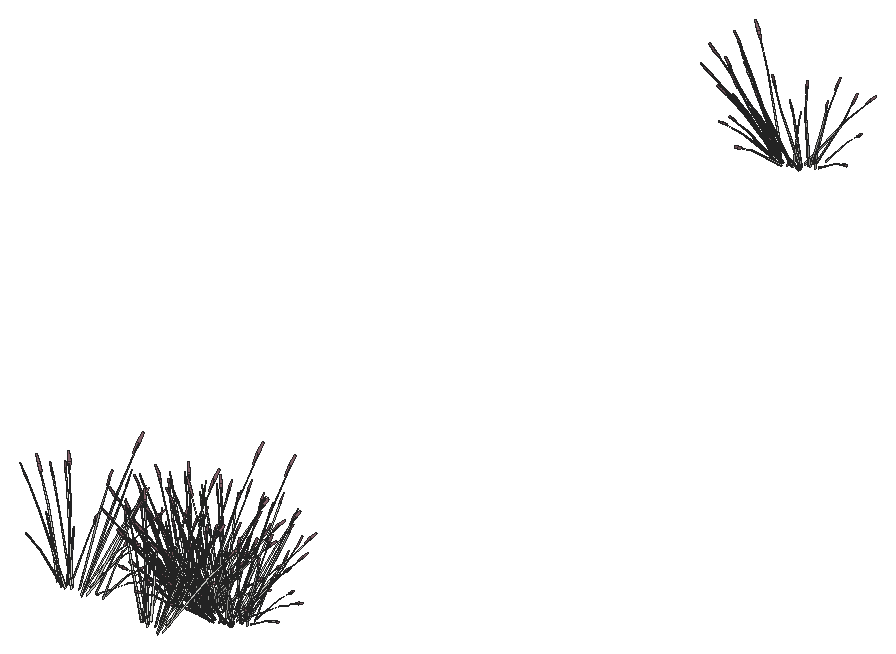
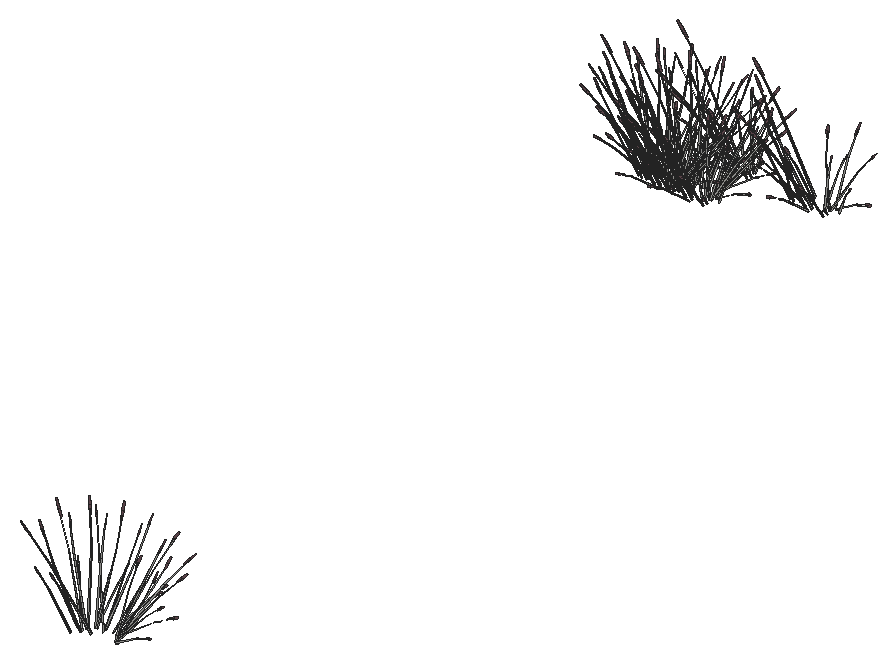
# SketchUp Ruby script. Lengths in inches.
U = 1.inch
M = Sketchup.active_model
def pt(a) = Geom::Point3d.new(a.map { |v| v * U })
def face(e, loops, mat)
  f = e.add_face(loops[0].map { |a| pt(a) })
  loops[1..].each { |l| e.add_face(l.map { |a| pt(a) }).erase! }
  f.material = f.back_material = mat if mat
  f
end
# faces: each face lists its corners as indices into pts; further lists are holes
def faces(e, pts, list, mat = nil) = list.each { |f| face(e, (f[0].is_a?(Array) ? f : [f]).map { |l| l.map { |i| pts[i] } }, mat) }
# xy, xz, yz: faces in a plane at the given z, y or x. An outline is a flat list of corners, or four numbers for a rectangle; further outlines are holes
def ring(l) = l.size == 4 ? [[l[0], l[1]], [l[2], l[1]], [l[2], l[3]], [l[0], l[3]]] : l.each_slice(2).to_a
def flat(e, list, mat, &to3) = list.each { |f| face(e, (f[0].is_a?(Array) ? f : [f]).map { |l| ring(l).map { |u, v| to3.(u, v) } }, mat) }
def xy(e, z, list, mat = nil) = flat(e, list, mat) { |x, y| [x, y, z] }
def xz(e, y, list, mat = nil) = flat(e, list, mat) { |x, z| [x, y, z] }
def yz(e, x, list, mat = nil) = flat(e, list, mat) { |y, z| [x, y, z] }
def lines(e, pts, list) = list.each { |a, b| e.add_line(pt(pts[a]), pt(pts[b])) }
# prism: a flat outline (further loops are holes) pulled along v
def prism(e, loops, v, mat = nil)
  f = face(e, loops, mat); d = Geom::Vector3d.new(v.map { |x| x * U })
  f.pushpull(f.normal.samedirection?(d) ? d.length : -d.length)
end
def box(e, o, s, mat = nil) = prism(e, [[o, [o[0] + s[0], o[1], o[2]], [o[0] + s[0], o[1] + s[1], o[2]], [o[0], o[1] + s[1], o[2]]]], [0, 0, s[2]], mat)
def at(x, y, z, deg = 0) = Geom::Transformation.translation(pt([x, y, z])) * Geom::Transformation.rotation(ORIGIN, Z_AXIS, deg.degrees)
def axes(o, x, y, z) = Geom::Transformation.new([*x, 0, *y, 0, *z, 0, *pt(o).to_a, 1])
def part(name) = M.definitions.add(name)
# library, detail: a bought-in or finely detailed component or shape, given as its bounding box
def library(name, o, s) = part(name).tap { |d| box(d.entities, o, s) }
def detail(e, o, s) = box(e.add_group.entities, o, s)
def put(e, d, t, mat = nil) = e.add_instance(d, t).tap { |i| i.material = mat if mat }
def group(e, t, mat = nil) = e.add_group.tap { |g| g.transformation = t; g.material = mat if mat }.entities
root = M.entities
M.materials.add("LightPink_Translucent").color = [144, 107, 117]
c1 = part("blade")
p = [[2.15,0.21,22],[0,0.17,0],[0.09,0.45,0],[2.18,0.31,22],[2.29,0.31,22],[0.38,0.45,0],
  [2.48,0.24,33],[2.49,0.24,33],[2.48,0.22,33]]
faces(c1.entities,p,[[0,1,2,3],[4,5,2,3],[6,3,4,7],[8,0,3,6]])
c2 = part("seeds")
p = [[0.3,-0.1,1.38],[-0.01,-0.03,1.59],[-0.01,-0.03,0.03],[0.14,-0.07,-0.07],[0.29,-0.03,3],[0.15,0.01,3.11]]
faces(c2.entities,p,[[0,1,2,3],[1,0,4,5]],"LightPink_Translucent")
c3 = part("blade with seeds")
put(c3.entities,c1,at(0,0,0))
put(c3.entities,c2,axes([2.4,0.25,30.99],[1.5799,-0.05474,1.17369],[-0.12525,1.92788,0.29478],[-0.07173,-0.02425,1.56792]))
put(root,c3,axes([57.68,55.28,46.53],[-1.06674,0.14801,-0.35414],[-0.28168,-0.84611,0.4572],[-0.30569,0.22726,0.87481]))
put(root,c3,axes([39.52,61.1,46.71],[-0.11081,-0.09067,1.77383],[0.2424,-0.97188,-0.16761],[0.43649,-0.06209,0.31391]))
put(root,c3,axes([25.1,57.15,46.72],[-0.20012,0.13446,1.74944],[0.01702,0.98243,-0.27667],[-0.45871,0.12776,0.14031]))
put(root,c3,axes([26.39,56.22,47.03],[0.6166,0.93779,-0.1216],[-1.09436,0.46085,-0.67495],[-0.46117,0.12373,1.02557]))
put(root,c3,axes([38.56,60.29,45.93],[-0.23455,-0.87059,-0.03492],[1.10861,-0.20015,-0.15832],[0.23151,0.05519,0.52218]))
put(root,c3,axes([35.69,60.26,47.03],[0.06562,-1.05324,-0.1216],[1.2424,0.02879,-0.67495],[0.4785,0.07316,1.02557]))
put(root,c3,axes([65.54,54.78,45.875],[-0.45521,-0.17844,1.71376],[0.94204,-0.74856,0.13857],[0.58713,0.33769,0.73262]))
put(root,c3,axes([65.63,52.43,46.47],[-1.05895,-0.53811,1.38283],[1.11816,-0.83781,0.59665],[0.34166,0.5049,1.33663]))
put(root,c3,axes([58,54.7,47.03],[1.1336,0.57106,-0.1216],[-0.65308,0.827,-0.67495],[-0.32027,0.28747,1.02557]))
put(root,c3,axes([64.8,57.66,47.03],[0.73026,-0.88648,-0.1216],[1.05755,0.51071,-0.67495],[0.36761,0.25045,1.02557]))
put(root,c3,axes([60.59,70.02,45.875],[0.28013,0.33252,1.71376],[-1.29445,0.27994,0.13857],[-0.29256,-0.52202,0.73262]))
put(root,c3,axes([72.59,70.02,45.875],[0.28013,0.33252,1.71376],[-1.29445,0.27994,0.13857],[-0.29256,-0.52202,0.73262]))
put(root,c3,axes([59.52,54.45,45.875],[0.30609,-0.31822,1.71376],[0.77286,0.85893,0.13857],[-0.53009,0.39116,0.73262]))
put(root,c3,axes([62.73,67.82,46.72],[-0.18744,-0.14521,1.74944],[-1.25089,0.09206,-0.27667],[-0.19964,-0.34731,0.14031]))
put(root,c3,axes([74.73,67.82,46.72],[-0.18744,-0.14521,1.74944],[-1.25089,0.09206,-0.27667],[-0.19964,-0.34731,0.14031]))
put(root,c3,axes([36.77,59.63,46.72],[0.26289,-0.01751,1.74944],[0.72108,-0.8046,-0.27667],[0.46761,0.10621,0.14031]))
put(root,c3,axes([26.4,57.51,45.875],[0.42521,-0.21906,1.71376],[0.35798,1.01226,0.13857],[-0.66754,0.22878,0.73262]))
put(root,c3,axes([63.85,58.4,46.71],[0.00363,-0.12539,1.77383],[1.0502,-0.55319,-0.16761],[0.36479,0.19745,0.31391]))
put(root,c3,axes([68.35,69.6,46.72],[-0.01183,-0.20612,1.74944],[-0.99913,-0.59572,-0.27667],[0.15447,-0.36112,0.14031]))
put(root,c3,axes([80.35,69.6,46.72],[-0.01183,-0.20612,1.74944],[-0.99913,-0.59572,-0.27667],[0.15447,-0.36112,0.14031]))
put(root,c3,axes([64.15,69.55,46.53],[0.36946,-0.79643,-0.35414],[1.07787,0.23229,0.4572],[-0.09883,-0.32066,0.87481]))
put(root,c3,axes([76.15,69.55,46.53],[0.36946,-0.79643,-0.35414],[1.07787,0.23229,0.4572],[-0.09883,-0.32066,0.87481]))
put(root,c3,axes([64.96,70.61,45.875],[-0.22818,0.35597,1.71376],[-0.95725,-0.73667,0.13857],[0.43183,-0.45914,0.73262]))
put(root,c3,axes([76.96,70.61,45.875],[-0.22818,0.35597,1.71376],[-0.95725,-0.73667,0.13857],[0.43183,-0.45914,0.73262]))
put(root,c3,axes([68.08,68.86,46.71],[-0.12446,0.07911,1.77383],[-1.21937,-0.26689,-0.16761],[-0.04414,-0.34521,0.31391]))
put(root,c3,axes([80.08,68.86,46.71],[-0.12446,0.07911,1.77383],[-1.21937,-0.26689,-0.16761],[-0.04414,-0.34521,0.31391]))
put(root,c3,axes([22.875,58.15,46.71],[0.1564,0.02778,1.77383],[0.48382,0.91506,-0.16761],[-0.32016,0.24017,0.31391]))
put(root,c3,axes([59.29,55.23,45.875],[0.22818,-0.35597,1.71376],[0.95725,0.73667,0.13857],[-0.43183,0.45914,0.73262]))
put(root,c3,axes([61.44,67.34,46.71],[-0.02286,0.12414,1.77383],[-1.12758,0.45052,-0.16761],[-0.33182,-0.23029,0.31391]))
put(root,c3,axes([73.44,67.34,46.71],[-0.02286,0.12414,1.77383],[-1.12758,0.45052,-0.16761],[-0.33182,-0.23029,0.31391]))
put(root,c3,axes([59.55,57.24,46.53],[-0.82919,0.54528,-0.35414],[-0.78493,-0.62262,0.4572],[-0.11943,0.31634,0.87481]))
put(root,c3,axes([56.7,57.08,46.72],[-0.03046,0.20495,1.74944],[0.86449,0.71297,-0.27667],[-0.22632,0.33716,0.14031]))
put(root,c3,axes([61.95,57.7,47.03],[1.19922,-0.48218,-0.1216],[0.58932,0.85579,-0.67495],[0.15822,0.36063,1.02557]))
put(root,c3,axes([64.63,70.06,47.03],[-1.19922,0.48218,-0.1216],[-0.58932,-0.85579,-0.67495],[-0.15822,-0.36063,1.02557]))
put(root,c3,axes([76.63,70.06,47.03],[-1.19922,0.48218,-0.1216],[-0.58932,-0.85579,-0.67495],[-0.15822,-0.36063,1.02557]))
put(root,c3,axes([67.12,71.14,47.03],[-1.34686,-0.05131,-0.1216],[0.03681,-0.97156,-0.67495],[0.09356,-0.37418,1.02557]))
put(root,c3,axes([79.12,71.14,47.03],[-1.34686,-0.05131,-0.1216],[0.03681,-0.97156,-0.67495],[0.09356,-0.37418,1.02557]))
put(root,c3,axes([67.03,70.52,46.53],[0.82919,-0.54528,-0.35414],[0.78493,0.62262,0.4572],[0.11943,-0.31634,0.87481]))
put(root,c3,axes([79.03,70.52,46.53],[0.82919,-0.54528,-0.35414],[0.78493,0.62262,0.4572],[0.11943,-0.31634,0.87481]))
put(root,c3,axes([33.98,58.52,45.875],[-0.45521,-0.17844,1.71376],[0.94204,-0.74856,0.13857],[0.58713,0.33769,0.73262]))
put(root,c3,axes([61.04,69.84,46.53],[-0.18927,-0.83419,-0.35414],[1.08199,-0.22027,0.4572],[-0.29062,-0.23905,0.87481]))
put(root,c3,axes([73.04,69.84,46.53],[-0.18927,-0.83419,-0.35414],[1.08199,-0.22027,0.4572],[-0.29062,-0.23905,0.87481]))
put(root,c3,axes([34.07,56.17,46.47],[-1.05895,-0.53811,1.38283],[1.11816,-0.83781,0.59665],[0.34166,0.5049,1.33663]))
put(root,c3,axes([26.43,58.45,47.03],[1.1336,0.57106,-0.1216],[-0.65308,0.827,-0.67495],[-0.32027,0.28747,1.02557]))
put(root,c3,axes([63.66,55.82,45.875],[-0.28013,-0.33252,1.71376],[1.29445,-0.27994,0.13857],[0.29256,0.52202,0.73262]))
put(root,c3,axes([33.24,61.41,47.03],[0.73026,-0.88648,-0.1216],[1.05755,0.51071,-0.67495],[0.36761,0.25045,1.02557]))
put(root,c3,axes([27.96,58.19,45.875],[0.30609,-0.31822,1.71376],[0.77286,0.85893,0.13857],[-0.53009,0.39116,0.73262]))
put(root,c3,axes([62.43,58.2,46.53],[-0.36946,0.79643,-0.35414],[-1.07787,-0.23229,0.4572],[0.09883,0.32066,0.87481]))
put(root,c3,axes([58.71,71.06,45.875],[0.45521,0.17844,1.71376],[-0.94204,0.74856,0.13857],[-0.58713,-0.33769,0.73262]))
put(root,c3,axes([70.71,71.06,45.875],[0.45521,0.17844,1.71376],[-0.94204,0.74856,0.13857],[-0.58713,-0.33769,0.73262]))
put(root,c3,axes([32.28,62.14,46.71],[0.00363,-0.12539,1.77383],[1.0502,-0.55319,-0.16761],[0.36479,0.19745,0.31391]))
put(root,c3,axes([56.6,59.18,46.71],[0.13903,-0.06253,1.77383],[1.14912,0.41591,-0.16761],[-0.027,0.34629,0.31391]))
put(root,c3,axes([61.38,55.98,45.875],[-0.02999,-0.3975,1.71376],[1.30002,0.26369,0.13857],[-0.08041,0.56647,0.73262]))
put(root,c3,axes([61.67,59.61,46.72],[0.15534,0.16677,1.74944],[1.25362,0.06552,-0.27667],[0.12606,0.3678,0.14031]))
put(root,c3,axes([58.625,69.41,46.72],[-0.26368,-0.00731,1.74944],[-0.83946,0.73103,-0.27667],[-0.44791,-0.14937,0.14031]))
put(root,c3,axes([70.625,69.41,46.72],[-0.26368,-0.00731,1.74944],[-0.83946,0.73103,-0.27667],[-0.44791,-0.14937,0.14031]))
put(root,c3,axes([68.59,73.05,47.03],[-1.1336,-0.57106,-0.1216],[0.65308,-0.827,-0.67495],[0.32027,-0.28747,1.02557]))
put(root,c3,axes([80.59,73.05,47.03],[-1.1336,-0.57106,-0.1216],[0.65308,-0.827,-0.67495],[0.32027,-0.28747,1.02557]))
put(root,c3,axes([27.73,58.97,45.875],[0.22818,-0.35597,1.71376],[0.95725,0.73667,0.13857],[-0.43183,0.45914,0.73262]))
put(root,c3,axes([25.13,60.82,46.72],[-0.03046,0.20495,1.74944],[0.86449,0.71297,-0.27667],[-0.22632,0.33716,0.14031]))
put(root,c3,axes([30.39,61.44,47.03],[1.19922,-0.48218,-0.1216],[0.58932,0.85579,-0.67495],[0.15822,0.36063,1.02557]))
put(root,c3,axes([71.38,72.8,46.71],[-0.16006,-0.00787,1.77383],[-0.66468,-0.8428,-0.16761],[0.26693,-0.27711,0.31391]))
put(root,c3,axes([83.38,72.8,46.71],[-0.16006,-0.00787,1.77383],[-0.66468,-0.8428,-0.16761],[0.26693,-0.27711,0.31391]))
put(root,c3,axes([68.9,72.48,46.53],[1.06674,-0.14801,-0.35414],[0.28168,0.84611,0.4572],[0.30569,-0.22726,0.87481]))
put(root,c3,axes([80.9,72.48,46.53],[1.06674,-0.14801,-0.35414],[0.28168,0.84611,0.4572],[0.30569,-0.22726,0.87481]))
put(root,c3,axes([32.1,59.5625,45.875],[-0.28013,-0.33252,1.71376],[1.29445,-0.27994,0.13857],[0.29256,0.52202,0.73262]))
put(root,c3,axes([58.54,71.3125,46.53],[-0.69728,-0.64842,-0.35414],[0.79619,-0.61382,0.4572],[-0.40453,-0.09339,0.87481]))
put(root,c3,axes([70.54,71.3125,46.53],[-0.69728,-0.64842,-0.35414],[0.79619,-0.61382,0.4572],[-0.40453,-0.09339,0.87481]))
put(root,c3,axes([25.04,62.92,46.71],[0.13903,-0.06253,1.77383],[1.14912,0.41591,-0.16761],[-0.027,0.34629,0.31391]))
put(root,c3,axes([29.82,59.73,45.875],[-0.02999,-0.3975,1.71376],[1.30002,0.26369,0.13857],[-0.08041,0.56647,0.73262]))
put(root,c3,axes([71.98,73.8125,46.72],[0.17006,-0.15775,1.74944],[-0.21766,-0.96766,-0.27667],[0.42669,-0.18347,0.14031]))
put(root,c3,axes([83.98,73.8125,46.72],[0.17006,-0.15775,1.74944],[-0.21766,-0.96766,-0.27667],[0.42669,-0.18347,0.14031]))
put(root,c3,axes([30.11,63.36,46.72],[0.15534,0.16677,1.74944],[1.25362,0.06552,-0.27667],[0.12606,0.3678,0.14031]))
put(root,c3,axes([57.61,70.03,46.71],[0.09085,0.10335,1.77383],[-0.43798,0.92907,-0.16761],[-0.44357,0.00672,0.31391]))
put(root,c3,axes([69.61,70.03,46.71],[0.09085,0.10335,1.77383],[-0.43798,0.92907,-0.16761],[-0.44357,0.00672,0.31391]))
put(root,c3,axes([59.33,71.24,47.03],[-0.06562,1.05324,-0.1216],[-1.2424,-0.02879,-0.67495],[-0.4785,-0.07316,1.02557]))
put(root,c3,axes([71.33,71.24,47.03],[-0.06562,1.05324,-0.1216],[-1.2424,-0.02879,-0.67495],[-0.4785,-0.07316,1.02557]))
put(root,c3,axes([68.63,75.28,47.03],[-0.6166,-0.93779,-0.1216],[1.09436,-0.46085,-0.67495],[0.46117,-0.12373,1.02557]))
put(root,c3,axes([80.63,75.28,47.03],[-0.6166,-0.93779,-0.1216],[1.09436,-0.46085,-0.67495],[0.46117,-0.12373,1.02557]))
put(root,c3,axes([57.75,72.69,45.875],[0.50831,-0.02346,1.71376],[-0.33721,1.01661,0.13857],[-0.72439,-0.06288,0.73262]))
put(root,c3,axes([69.75,72.69,45.875],[0.50831,-0.02346,1.71376],[-0.33721,1.01661,0.13857],[-0.72439,-0.06288,0.73262]))
put(root,c3,axes([69.28,74.91,46.53],[1.01846,0.28891,-0.35414],[-0.29705,0.84289,0.4572],[0.41005,-0.07729,0.87481]))
put(root,c3,axes([81.28,74.91,46.53],[1.01846,0.28891,-0.35414],[-0.29705,0.84289,0.4572],[0.41005,-0.07729,0.87481]))
put(root,c3,axes([57.31,73.5625,46.53],[-1.01846,-0.28891,-0.35414],[0.29705,-0.84289,0.4572],[-0.41005,0.07729,0.87481]))
put(root,c3,axes([69.31,73.5625,46.53],[-1.01846,-0.28891,-0.35414],[0.29705,-0.84289,0.4572],[-0.41005,0.07729,0.87481]))
put(root,c3,axes([66.5,73.86,45.875],[-0.50831,0.02346,1.71376],[0.33721,-1.01661,0.13857],[0.72439,0.06288,0.73262]))
put(root,c3,axes([78.5,73.86,45.875],[-0.50831,0.02346,1.71376],[0.33721,-1.01661,0.13857],[0.72439,0.06288,0.73262]))
put(root,c3,axes([71.08,78.07,46.71],[-0.11081,-0.09067,1.77383],[0.2424,-0.97188,-0.16761],[0.43649,-0.06209,0.31391]))
put(root,c3,axes([83.08,78.07,46.71],[-0.11081,-0.09067,1.77383],[0.2424,-0.97188,-0.16761],[0.43649,-0.06209,0.31391]))
put(root,c3,axes([56.66,74.125,46.72],[-0.20012,0.13446,1.74944],[0.01702,0.98243,-0.27667],[-0.45871,0.12776,0.14031]))
put(root,c3,axes([68.66,74.125,46.72],[-0.20012,0.13446,1.74944],[0.01702,0.98243,-0.27667],[-0.45871,0.12776,0.14031]))
put(root,c3,axes([57.95,73.1875,47.03],[0.6166,0.93779,-0.1216],[-1.09436,0.46085,-0.67495],[-0.46117,0.12373,1.02557]))
put(root,c3,axes([69.95,73.1875,47.03],[0.6166,0.93779,-0.1216],[-1.09436,0.46085,-0.67495],[-0.46117,0.12373,1.02557]))
put(root,c3,axes([70.12,77.26,45.93],[-0.23455,-0.87059,-0.03492],[1.10861,-0.20015,-0.15832],[0.23151,0.05519,0.52218]))
put(root,c3,axes([82.12,77.26,45.93],[-0.23455,-0.87059,-0.03492],[1.10861,-0.20015,-0.15832],[0.23151,0.05519,0.52218]))
put(root,c3,axes([67.25,77.23,47.03],[0.06562,-1.05324,-0.1216],[1.2424,0.02879,-0.67495],[0.4785,0.07316,1.02557]))
put(root,c3,axes([79.25,77.23,47.03],[0.06562,-1.05324,-0.1216],[1.2424,0.02879,-0.67495],[0.4785,0.07316,1.02557]))
put(root,c3,axes([68.33,76.6,46.72],[0.26289,-0.01751,1.74944],[0.72108,-0.8046,-0.27667],[0.46761,0.10621,0.14031]))
put(root,c3,axes([80.33,76.6,46.72],[0.26289,-0.01751,1.74944],[0.72108,-0.8046,-0.27667],[0.46761,0.10621,0.14031]))
put(root,c3,axes([57.96,74.48,45.875],[0.42521,-0.21906,1.71376],[0.35798,1.01226,0.13857],[-0.66754,0.22878,0.73262]))
put(root,c3,axes([69.96,74.48,45.875],[0.42521,-0.21906,1.71376],[0.35798,1.01226,0.13857],[-0.66754,0.22878,0.73262]))
put(root,c3,axes([54.4375,75.12,46.71],[0.1564,0.02778,1.77383],[0.48382,0.91506,-0.16761],[-0.32016,0.24017,0.31391]))
put(root,c3,axes([66.4375,75.12,46.71],[0.1564,0.02778,1.77383],[0.48382,0.91506,-0.16761],[-0.32016,0.24017,0.31391]))
put(root,c3,axes([68.05,77.16,46.53],[0.69728,0.64842,-0.35414],[-0.79619,0.61382,0.4572],[0.40453,0.09339,0.87481]))
put(root,c3,axes([80.05,77.16,46.53],[0.69728,0.64842,-0.35414],[-0.79619,0.61382,0.4572],[0.40453,0.09339,0.87481]))
put(root,c3,axes([57.68,75.99,46.53],[-1.06674,0.14801,-0.35414],[-0.28168,-0.84611,0.4572],[-0.30569,0.22726,0.87481]))
put(root,c3,axes([69.68,75.99,46.53],[-1.06674,0.14801,-0.35414],[-0.28168,-0.84611,0.4572],[-0.30569,0.22726,0.87481]))
put(root,c3,axes([65.54,75.49,45.875],[-0.45521,-0.17844,1.71376],[0.94204,-0.74856,0.13857],[0.58713,0.33769,0.73262]))
put(root,c3,axes([77.54,75.49,45.875],[-0.45521,-0.17844,1.71376],[0.94204,-0.74856,0.13857],[0.58713,0.33769,0.73262]))
put(root,c3,axes([65.63,73.14,46.47],[-1.05895,-0.53811,1.38283],[1.11816,-0.83781,0.59665],[0.34166,0.5049,1.33663]))
put(root,c3,axes([77.63,73.14,46.47],[-1.05895,-0.53811,1.38283],[1.11816,-0.83781,0.59665],[0.34166,0.5049,1.33663]))
put(root,c3,axes([58,75.42,47.03],[1.1336,0.57106,-0.1216],[-0.65308,0.827,-0.67495],[-0.32027,0.28747,1.02557]))
put(root,c3,axes([70,75.42,47.03],[1.1336,0.57106,-0.1216],[-0.65308,0.827,-0.67495],[-0.32027,0.28747,1.02557]))
put(root,c3,axes([64.8,78.375,47.03],[0.73026,-0.88648,-0.1216],[1.05755,0.51071,-0.67495],[0.36761,0.25045,1.02557]))
put(root,c3,axes([76.8,78.375,47.03],[0.73026,-0.88648,-0.1216],[1.05755,0.51071,-0.67495],[0.36761,0.25045,1.02557]))
put(root,c3,axes([59.52,75.16,45.875],[0.30609,-0.31822,1.71376],[0.77286,0.85893,0.13857],[-0.53009,0.39116,0.73262]))
put(root,c3,axes([71.52,75.16,45.875],[0.30609,-0.31822,1.71376],[0.77286,0.85893,0.13857],[-0.53009,0.39116,0.73262]))
put(root,c3,axes([63.85,79.11,46.71],[0.00363,-0.12539,1.77383],[1.0502,-0.55319,-0.16761],[0.36479,0.19745,0.31391]))
put(root,c3,axes([75.85,79.11,46.71],[0.00363,-0.12539,1.77383],[1.0502,-0.55319,-0.16761],[0.36479,0.19745,0.31391]))
put(root,c3,axes([59.29,75.95,45.875],[0.22818,-0.35597,1.71376],[0.95725,0.73667,0.13857],[-0.43183,0.45914,0.73262]))
put(root,c3,axes([71.29,75.95,45.875],[0.22818,-0.35597,1.71376],[0.95725,0.73667,0.13857],[-0.43183,0.45914,0.73262]))
put(root,c3,axes([59.55,77.95,46.53],[-0.82919,0.54528,-0.35414],[-0.78493,-0.62262,0.4572],[-0.11943,0.31634,0.87481]))
put(root,c3,axes([71.55,77.95,46.53],[-0.82919,0.54528,-0.35414],[-0.78493,-0.62262,0.4572],[-0.11943,0.31634,0.87481]))
put(root,c3,axes([56.7,77.79,46.72],[-0.03046,0.20495,1.74944],[0.86449,0.71297,-0.27667],[-0.22632,0.33716,0.14031]))
put(root,c3,axes([68.7,77.79,46.72],[-0.03046,0.20495,1.74944],[0.86449,0.71297,-0.27667],[-0.22632,0.33716,0.14031]))
put(root,c3,axes([61.95,78.41,47.03],[1.19922,-0.48218,-0.1216],[0.58932,0.85579,-0.67495],[0.15822,0.36063,1.02557]))
put(root,c3,axes([73.95,78.41,47.03],[1.19922,-0.48218,-0.1216],[0.58932,0.85579,-0.67495],[0.15822,0.36063,1.02557]))
put(root,c3,axes([63.66,76.53,45.875],[-0.28013,-0.33252,1.71376],[1.29445,-0.27994,0.13857],[0.29256,0.52202,0.73262]))
put(root,c3,axes([75.66,76.53,45.875],[-0.28013,-0.33252,1.71376],[1.29445,-0.27994,0.13857],[0.29256,0.52202,0.73262]))
put(root,c3,axes([62.43,78.91,46.53],[-0.36946,0.79643,-0.35414],[-1.07787,-0.23229,0.4572],[0.09883,0.32066,0.87481]))
put(root,c3,axes([74.43,78.91,46.53],[-0.36946,0.79643,-0.35414],[-1.07787,-0.23229,0.4572],[0.09883,0.32066,0.87481]))
put(root,c3,axes([56.6,79.89,46.71],[0.13903,-0.06253,1.77383],[1.14912,0.41591,-0.16761],[-0.027,0.34629,0.31391]))
put(root,c3,axes([68.6,79.89,46.71],[0.13903,-0.06253,1.77383],[1.14912,0.41591,-0.16761],[-0.027,0.34629,0.31391]))
put(root,c3,axes([61.38,76.7,45.875],[-0.02999,-0.3975,1.71376],[1.30002,0.26369,0.13857],[-0.08041,0.56647,0.73262]))
put(root,c3,axes([73.38,76.7,45.875],[-0.02999,-0.3975,1.71376],[1.30002,0.26369,0.13857],[-0.08041,0.56647,0.73262]))
put(root,c3,axes([61.67,80.33,46.72],[0.15534,0.16677,1.74944],[1.25362,0.06552,-0.27667],[0.12606,0.3678,0.14031]))
put(root,c3,axes([73.67,80.33,46.72],[0.15534,0.16677,1.74944],[1.25362,0.06552,-0.27667],[0.12606,0.3678,0.14031]))
put(root,c3,axes([31.75,388.76,45.875],[0.28013,0.33252,1.71376],[-1.29445,0.27994,0.13857],[-0.29256,-0.52202,0.73262]))
put(root,c3,axes([33.89,386.56,46.72],[-0.18744,-0.14521,1.74944],[-1.25089,0.09206,-0.27667],[-0.19964,-0.34731,0.14031]))
put(root,c3,axes([39.51,388.34,46.72],[-0.01183,-0.20612,1.74944],[-0.99913,-0.59572,-0.27667],[0.15447,-0.36112,0.14031]))
put(root,c3,axes([35.31,388.29,46.53],[0.36946,-0.79643,-0.35414],[1.07787,0.23229,0.4572],[-0.09883,-0.32066,0.87481]))
put(root,c3,axes([36.12,389.35,45.875],[-0.22818,0.35597,1.71376],[-0.95725,-0.73667,0.13857],[0.43183,-0.45914,0.73262]))
put(root,c3,axes([39.24,387.59,46.71],[-0.12446,0.07911,1.77383],[-1.21937,-0.26689,-0.16761],[-0.04414,-0.34521,0.31391]))
put(root,c3,axes([32.6,386.08,46.71],[-0.02286,0.12414,1.77383],[-1.12758,0.45052,-0.16761],[-0.33182,-0.23029,0.31391]))
put(root,c3,axes([35.79,388.8,47.03],[-1.19922,0.48218,-0.1216],[-0.58932,-0.85579,-0.67495],[-0.15822,-0.36063,1.02557]))
put(root,c3,axes([38.28,389.88,47.03],[-1.34686,-0.05131,-0.1216],[0.03681,-0.97156,-0.67495],[0.09356,-0.37418,1.02557]))
put(root,c3,axes([38.1875,389.25,46.53],[0.82919,-0.54528,-0.35414],[0.78493,0.62262,0.4572],[0.11943,-0.31634,0.87481]))
put(root,c3,axes([32.2,388.58,46.53],[-0.18927,-0.83419,-0.35414],[1.08199,-0.22027,0.4572],[-0.29062,-0.23905,0.87481]))
put(root,c3,axes([29.875,389.8,45.875],[0.45521,0.17844,1.71376],[-0.94204,0.74856,0.13857],[-0.58713,-0.33769,0.73262]))
put(root,c3,axes([29.78,388.15,46.72],[-0.26368,-0.00731,1.74944],[-0.83946,0.73103,-0.27667],[-0.44791,-0.14937,0.14031]))
put(root,c3,axes([39.75,391.79,47.03],[-1.1336,-0.57106,-0.1216],[0.65308,-0.827,-0.67495],[0.32027,-0.28747,1.02557]))
put(root,c3,axes([42.54,391.54,46.71],[-0.16006,-0.00787,1.77383],[-0.66468,-0.8428,-0.16761],[0.26693,-0.27711,0.31391]))
put(root,c3,axes([40.0625,391.21,46.53],[1.06674,-0.14801,-0.35414],[0.28168,0.84611,0.4572],[0.30569,-0.22726,0.87481]))
put(root,c3,axes([29.7,390.05,46.53],[-0.69728,-0.64842,-0.35414],[0.79619,-0.61382,0.4572],[-0.40453,-0.09339,0.87481]))
put(root,c3,axes([43.14,392.55,46.72],[0.17006,-0.15775,1.74944],[-0.21766,-0.96766,-0.27667],[0.42669,-0.18347,0.14031]))
put(root,c3,axes([28.77,388.77,46.71],[0.09085,0.10335,1.77383],[-0.43798,0.92907,-0.16761],[-0.44357,0.00672,0.31391]))
put(root,c3,axes([30.49,389.98,47.03],[-0.06562,1.05324,-0.1216],[-1.2424,-0.02879,-0.67495],[-0.4785,-0.07316,1.02557]))
put(root,c3,axes([39.79,394.02,47.03],[-0.6166,-0.93779,-0.1216],[1.09436,-0.46085,-0.67495],[0.46117,-0.12373,1.02557]))
put(root,c3,axes([28.91,391.43,45.875],[0.50831,-0.02346,1.71376],[-0.33721,1.01661,0.13857],[-0.72439,-0.06288,0.73262]))
put(root,c3,axes([40.4375,393.64,46.53],[1.01846,0.28891,-0.35414],[-0.29705,0.84289,0.4572],[0.41005,-0.07729,0.87481]))
put(root,c3,axes([28.46,392.3,46.53],[-1.01846,-0.28891,-0.35414],[0.29705,-0.84289,0.4572],[-0.41005,0.07729,0.87481]))
put(root,c3,axes([37.66,392.6,45.875],[-0.50831,0.02346,1.71376],[0.33721,-1.01661,0.13857],[0.72439,0.06288,0.73262]))
put(root,c3,axes([42.24,396.81,46.71],[-0.11081,-0.09067,1.77383],[0.2424,-0.97188,-0.16761],[0.43649,-0.06209,0.31391]))
put(root,c3,axes([27.82,392.86,46.72],[-0.20012,0.13446,1.74944],[0.01702,0.98243,-0.27667],[-0.45871,0.12776,0.14031]))
put(root,c3,axes([29.11,391.93,47.03],[0.6166,0.93779,-0.1216],[-1.09436,0.46085,-0.67495],[-0.46117,0.12373,1.02557]))
